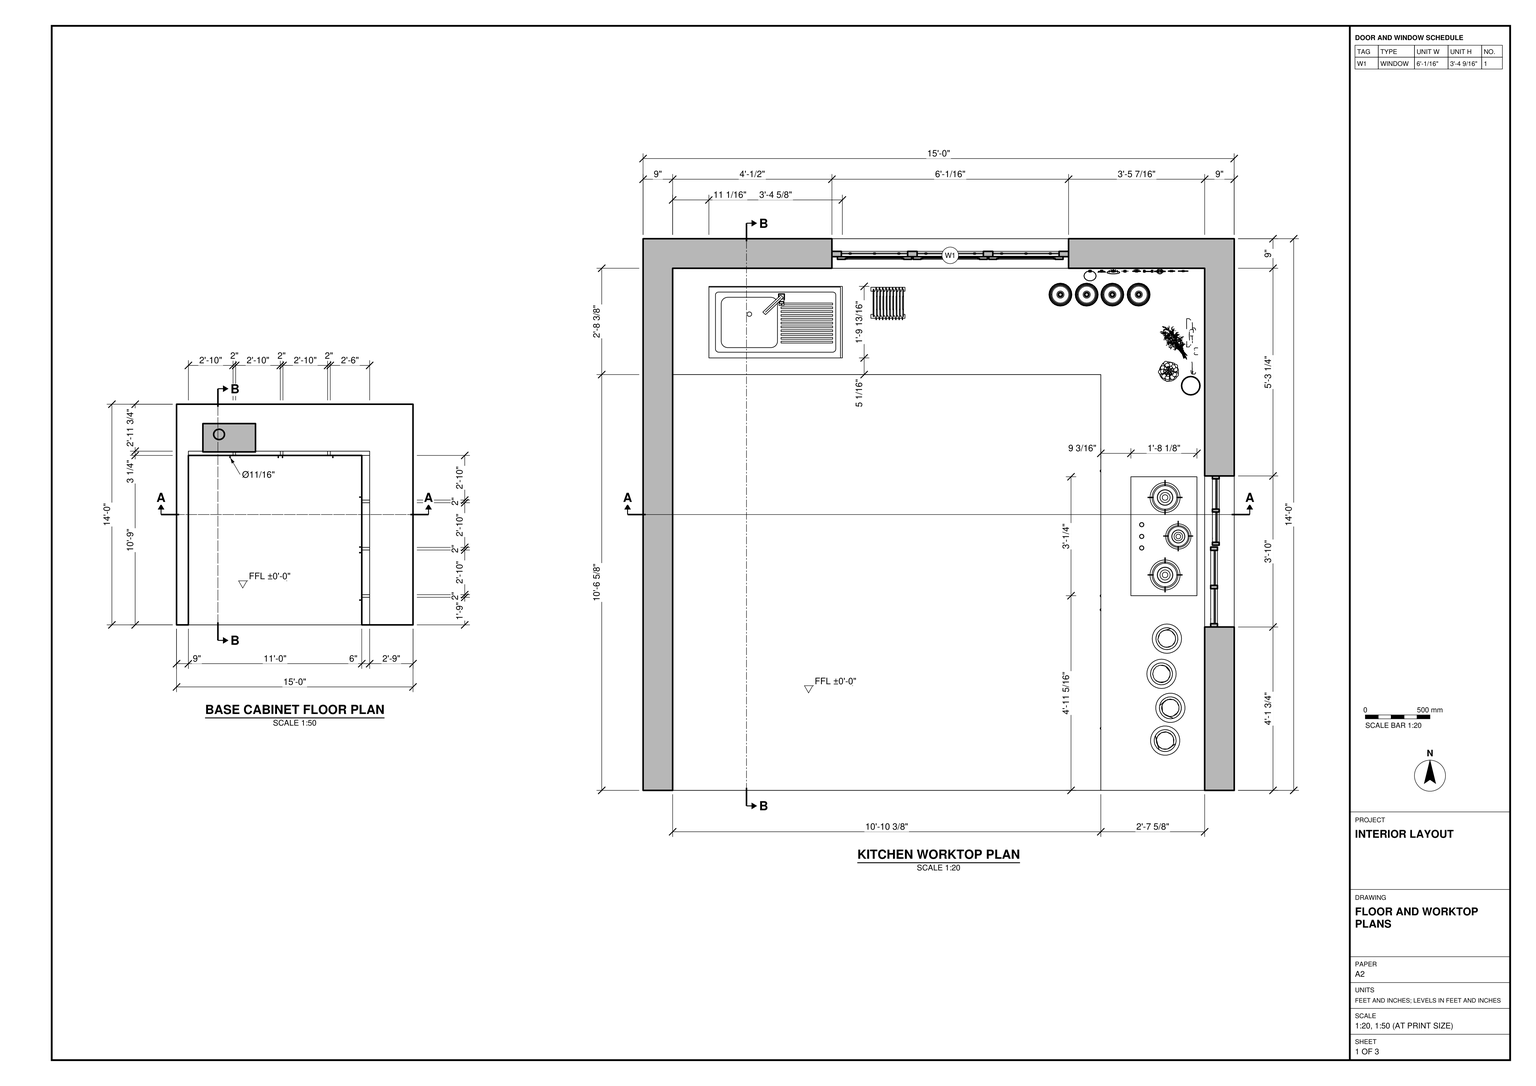
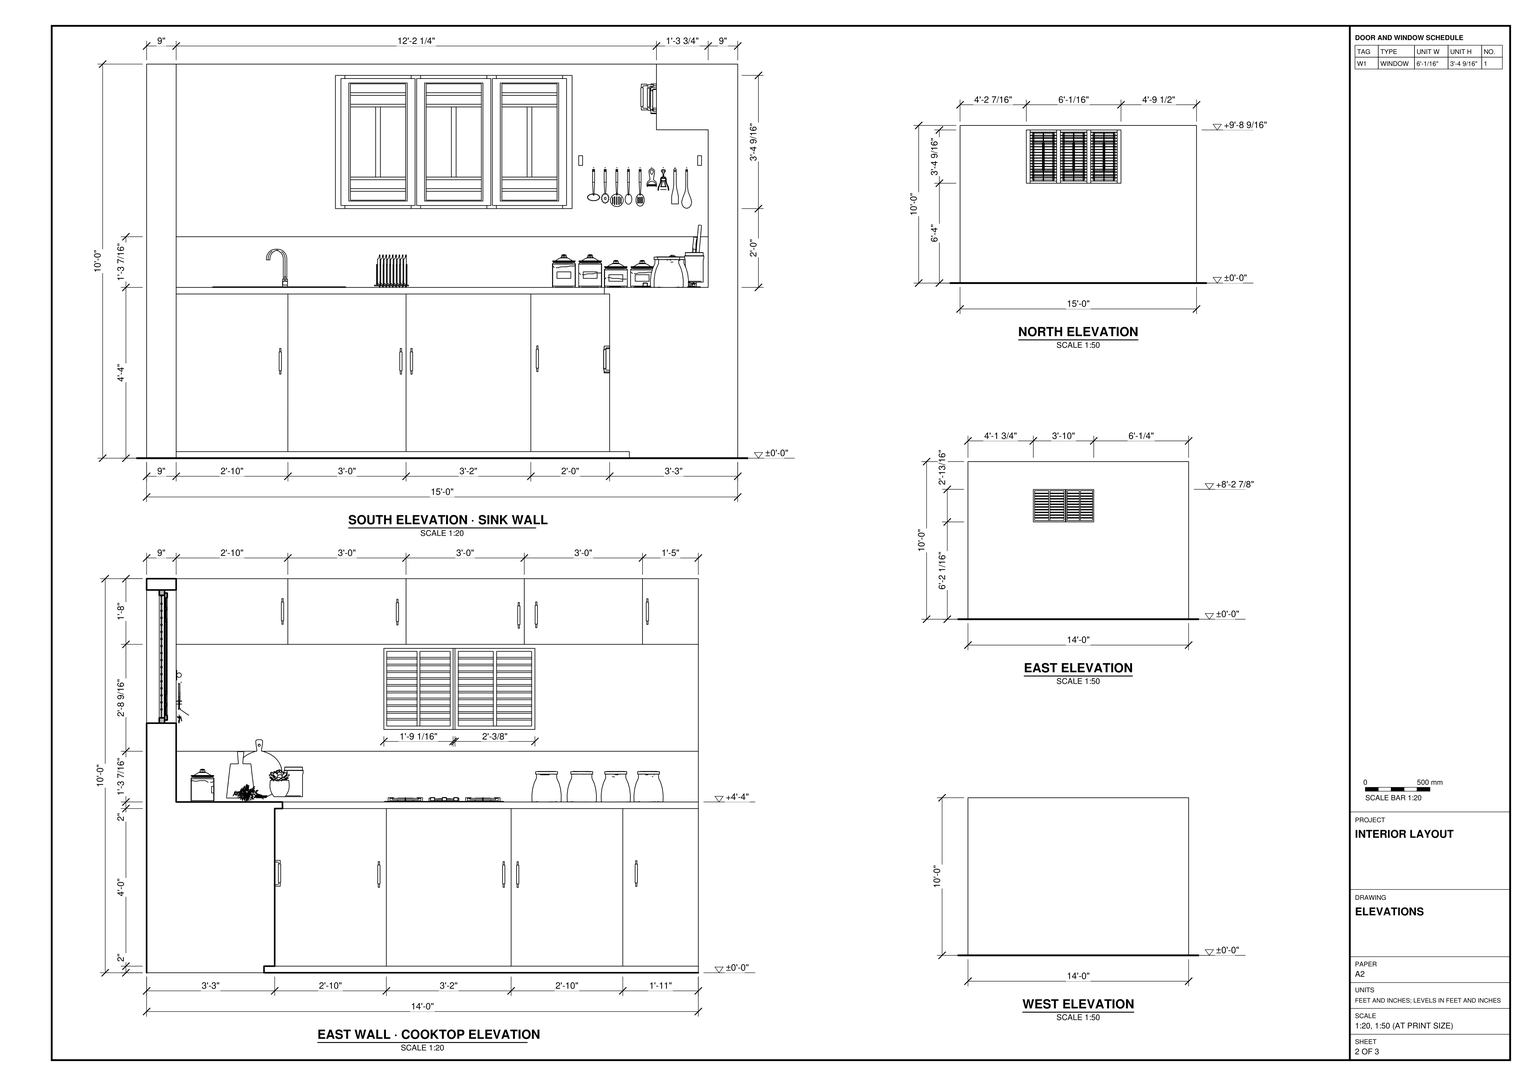
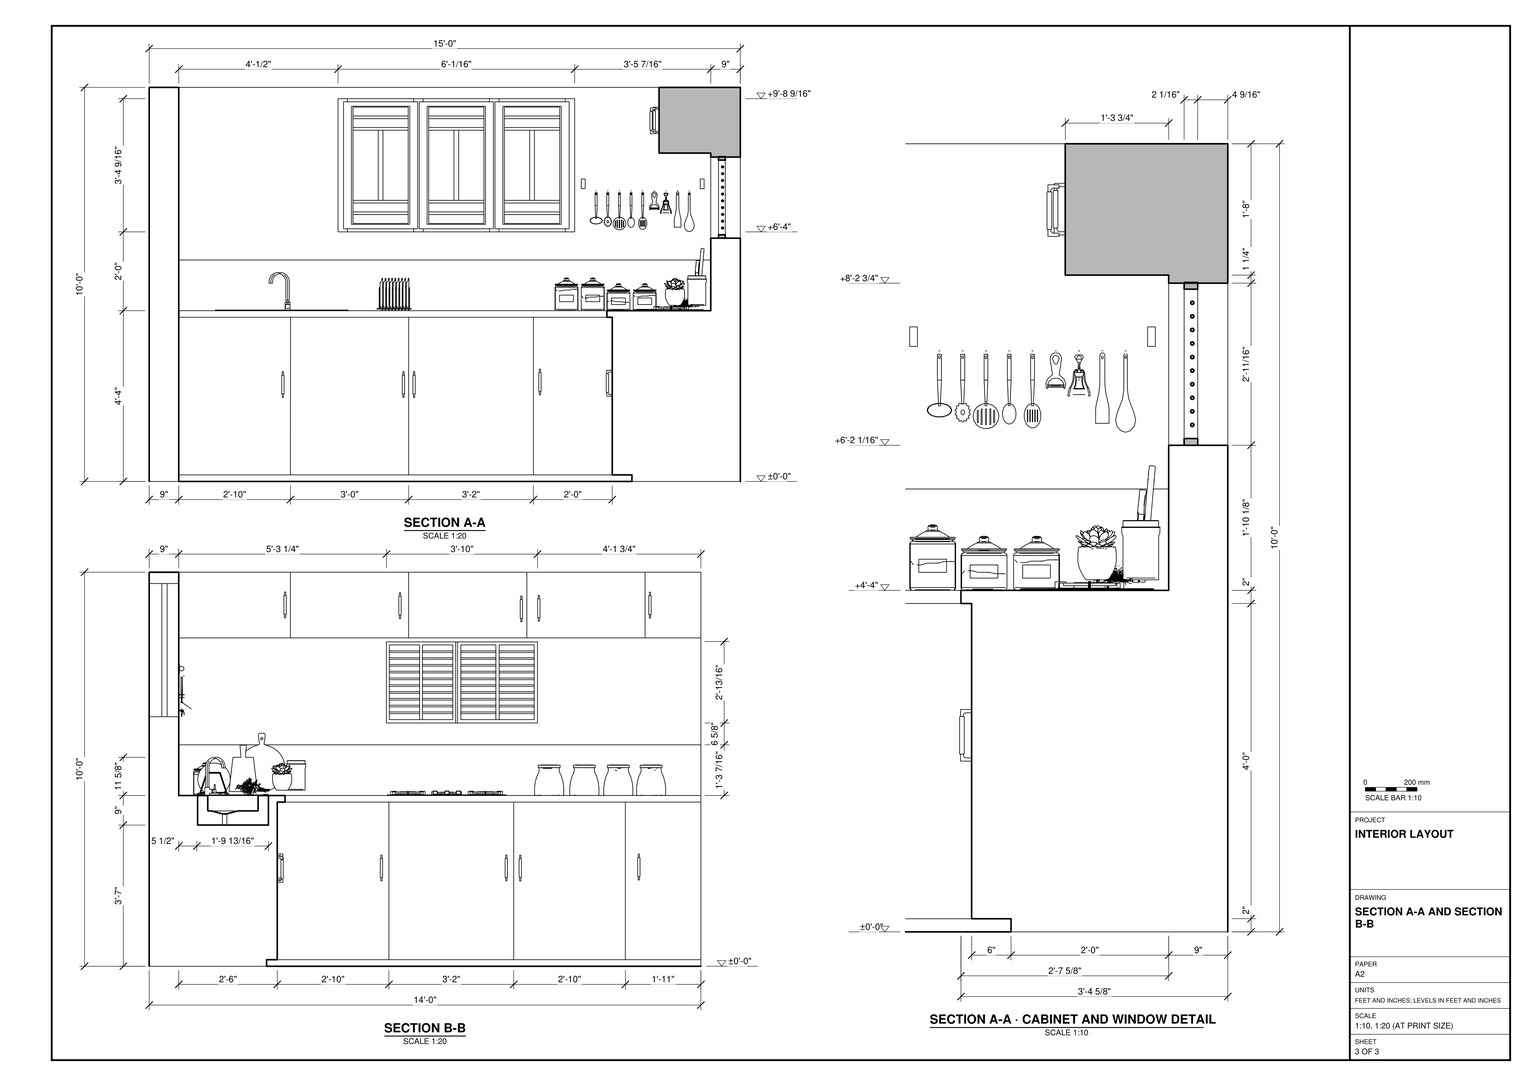
Build the kitchen interior in SketchUp from task_files/diagram_01.pdf. Work in feet and inches. Set the finished floor at ±0'-0" and make the overall model 15'-0" wide by 14'-0" deep by 10'-0" high. Model the floor and the 9" walls on the north, east and west sides, leaving the south side open as drawn. Use the plans to locate the openings and the elevations to set the sills and frames of the wide north window and smaller east window.

Fit a continuous L-shaped worktop along the north and east walls, with its top 4'-4" above the finished floor. Use the base cabinet plan for the cabinet divisions and the sections for the worktop edges and plinths. Place the sink toward the west end of the north run, with its tap and draining board, and fit the cooktop into the east return. Model the row of upper cabinets above the east window. Match the cabinet door widths and handle positions to the elevations.

Keep the floor, walls and each fitted joinery piece in separate groups or components, and use components for repeated parts. Decor, loose kitchen items and appliances may be any suitable library components placed as shown. Save one SketchUp model as output_files/l_shaped_kitchen_with_fitted_cabinets_and_window_units.skp.

# SketchUp Ruby script. Lengths in inches.
U = 1.inch
M = Sketchup.active_model
def pt(a) = Geom::Point3d.new(a.map { |v| v * U })
def face(e, loops, mat)
  f = e.add_face(loops[0].map { |a| pt(a) })
  loops[1..].each { |l| e.add_face(l.map { |a| pt(a) }).erase! }
  f.material = f.back_material = mat if mat
  f
end
# faces: each face lists its corners as indices into pts; further lists are holes
def faces(e, pts, list, mat = nil) = list.each { |f| face(e, (f[0].is_a?(Array) ? f : [f]).map { |l| l.map { |i| pts[i] } }, mat) }
# xy, xz, yz: faces in a plane at the given z, y or x. An outline is a flat list of corners, or four numbers for a rectangle; further outlines are holes
def ring(l) = l.size == 4 ? [[l[0], l[1]], [l[2], l[1]], [l[2], l[3]], [l[0], l[3]]] : l.each_slice(2).to_a
def flat(e, list, mat, &to3) = list.each { |f| face(e, (f[0].is_a?(Array) ? f : [f]).map { |l| ring(l).map { |u, v| to3.(u, v) } }, mat) }
def xy(e, z, list, mat = nil) = flat(e, list, mat) { |x, y| [x, y, z] }
def xz(e, y, list, mat = nil) = flat(e, list, mat) { |x, z| [x, y, z] }
def yz(e, x, list, mat = nil) = flat(e, list, mat) { |y, z| [x, y, z] }
def lines(e, pts, list) = list.each { |a, b| e.add_line(pt(pts[a]), pt(pts[b])) }
# prism: a flat outline (further loops are holes) pulled along v
def prism(e, loops, v, mat = nil)
  f = face(e, loops, mat); d = Geom::Vector3d.new(v.map { |x| x * U })
  f.pushpull(f.normal.samedirection?(d) ? d.length : -d.length)
end
def box(e, o, s, mat = nil) = prism(e, [[o, [o[0] + s[0], o[1], o[2]], [o[0] + s[0], o[1] + s[1], o[2]], [o[0], o[1] + s[1], o[2]]]], [0, 0, s[2]], mat)
def at(x, y, z, deg = 0) = Geom::Transformation.translation(pt([x, y, z])) * Geom::Transformation.rotation(ORIGIN, Z_AXIS, deg.degrees)
def axes(o, x, y, z) = Geom::Transformation.new([*x, 0, *y, 0, *z, 0, *pt(o).to_a, 1])
def part(name) = M.definitions.add(name)
# library, detail: a bought-in or finely detailed component or shape, given as its bounding box
def library(name, o, s) = part(name).tap { |d| box(d.entities, o, s) }
def detail(e, o, s) = box(e.add_group.entities, o, s)
def put(e, d, t, mat = nil) = e.add_instance(d, t).tap { |i| i.material = mat if mat }
def group(e, t, mat = nil) = e.add_group.tap { |g| g.transformation = t; g.material = mat if mat }.entities
root = M.entities
M.materials.add("[Cardboard]").color = [189, 139, 76]
M.materials.add("[Chipboard]").color = [205, 176, 119]
M.materials.add("[Color M08]").color = [30, 30, 30]
M.materials.add("[Encaustic Tile Circular 01]").color = [123, 123, 122]
M.materials.add("[Stone Vein Gray]").color = [166, 165, 165]
M.materials.add("[Translucent Glass Gray]").color = [128, 128, 128]
M.materials["[Translucent Glass Gray]"].alpha = 0.5
M.materials.add("[Wood Cherry Original]").color = [152, 86, 42]
M.materials.add("[Wood Floor Parquet]").color = [142, 87, 38]
M.materials.add("[Wood Veneer 01]").color = [120, 70, 37]
M.materials.add("[Wood Veneer 02]").color = [190, 128, 91]
c1 = library("w1.2X1.2",[0,0,0],[3.9375,47.24,47.24])
c2 = part("Group\#19")
box(c2.entities,[0,0,0],[13.78,1.18,1.18])
c3 = part("Group\#23")
box(c3.entities,[0,0.39,0],[13.78,0.4,3.9375])
c4 = part("Group\#21")
box(c4.entities,[0,0.39,0],[6.3,0.4,3.9375])
c5 = part("w3a")
g1 = group(c5.entities,at(-0.98,-1.18,-0.98),"[Wood Floor Parquet]")
xy(g1,0,[[0,0,18.5,1.18]])
xy(g1,1.97,[[1.97,0,16.54,0.39]])
xy(g1,2.36,[[2.36,0.39,16.14,1.18]])
xy(g1,53.9375,[[2.36,0.39,16.14,1.18]])
xy(g1,54.33,[[1.97,0,16.54,0.39]])
xy(g1,56.3,[[0,0,18.5,1.18]])
xz(g1,0,[[[0,0,18.5,56.3],[1.97,1.97,16.54,54.33]]])
xz(g1,0.39,[[[1.97,1.97,16.54,54.33],[2.36,2.36,16.14,53.9375]]])
xz(g1,1.18,[[[0,0,18.5,56.3],[2.36,2.36,16.14,53.9375]]])
yz(g1,0,[[0,0,1.18,56.3]])
yz(g1,1.97,[[0,1.97,0.39,54.33]])
yz(g1,2.36,[[0.39,2.36,1.18,53.9375]])
yz(g1,16.14,[[0.39,2.36,1.18,53.9375]])
yz(g1,16.54,[[0,1.97,0.39,54.33]])
yz(g1,18.5,[[0,0,1.18,56.3]])
g2 = group(c5.entities,at(1.38,-1.18,5.31),"[Wood Floor Parquet]")
put(g2,c2,axes([0,0.39,42.52],[1,0,0],[0,0.66667,0],[0,0,1]))
g3 = group(g2,at(6.3,0.39,20.08))
box(g3,[0,0,-13.78],[1.18,0.79,31.1])
put(g2,c2,axes([0,0.39,37.4],[1,0,0],[0,0.66667,0],[0,0,1]))
put(g2,c2,axes([0,0.39,0],[1,0,0],[0,0.66667,0],[0,0,1]))
put(g2,c2,axes([0,0.39,5.12],[1,0,0],[0,0.66667,0],[0,0,1]))
g4 = group(c5.entities,at(1.38,-0.39,1.38),"[Translucent Glass Gray]")
put(g4,c3,at(0,-0.39,5.12))
put(g4,c3,at(0,-0.39,0))
put(g4,c4,axes([0,-0.39,10.24],[1,0,0],[0,1,0],[0,0,7.9]))
put(g4,c4,axes([7.48,-0.39,10.24],[1,0,0],[0,1,0],[0,0,7.9]))
put(g4,c3,at(0,-0.39,47.64))
put(g4,c3,at(0,-0.39,42.52))
c6 = part("Group\#26")
box(c6.entities,[0,0,0],[0.39,0.39,54.33])
c7 = part("Group\#24")
box(c7.entities,[0,0,0],[0.39,0.39,5.68])
c8 = part("Group\#27")
box(c8.entities,[0,0,0],[0.39,0.39,2])
c9 = part("Group\#28")
put(c9.entities,c7,axes([14.14,0,0],[0,0,1],[0,1,0],[-1,0,0]))
put(c9.entities,c8,axes([2,0,0],[0,0,1],[0,1,0],[-1,0,0]))
put(c9.entities,c7,axes([8.07,0,0],[0,0,1],[0,1,0],[-1,0,0]))
put(c9.entities,c8,axes([16.54,0,0],[0,0,1],[0,1,0],[-1,0,0]))
c10 = part("Group\#29")
put(c10.entities,c6,at(12.15,0,0))
put(c10.entities,c6,at(6.07,0,0))
put(c10.entities,c6,at(0,0,0))
put(c10.entities,c9,at(-2,0,53.93))
put(c10.entities,c9,at(-2,0,50.39))
put(c10.entities,c9,at(-2,0,47.27))
put(c10.entities,c9,at(-2,0,44.14))
put(c10.entities,c9,at(-2,0,41.02))
put(c10.entities,c9,at(-2,0,37.9))
put(c10.entities,c9,at(-2,0,34.77))
put(c10.entities,c9,at(-2,0,31.65))
put(c10.entities,c9,at(-2,0,28.53))
put(c10.entities,c9,at(-2,0,25.4))
put(c10.entities,c9,at(-2,0,22.28))
put(c10.entities,c9,at(-2,0,19.16))
put(c10.entities,c9,at(-2,0,16.03))
put(c10.entities,c9,at(-2,0,12.91))
put(c10.entities,c9,at(-2,0,9.79))
put(c10.entities,c9,at(-2,0,6.66))
put(c10.entities,c9,at(-2,0,3.54))
c11 = part("Group\#16")
box(c11.entities,[0,0,0],[2.36,2.36,59.06])
c12 = part("Group\#1")
box(c12.entities,[0,0,0],[2.36,2.36,16.54])
c13 = part("W3")
put(c13.entities,c5,at(2.36,1.18,2.36))
put(c13.entities,c5,at(21.26,1.18,2.36))
put(c13.entities,c5,at(40.16,1.18,2.36))
put(c13.entities,c10,at(23.26,2.38,2.36),"[Color M08]")
put(c13.entities,c10,at(4.36,2.38,2.36),"[Color M08]")
put(c13.entities,c10,at(42.15,2.38,2.36),"[Color M08]")
g5 = group(c13.entities,at(0,1.18,0),"[Wood Veneer 01]")
put(g5,c11,at(0,0,0))
put(g5,c12,axes([2.36,0,2.36],[0,0,-1],[0,1,0],[1,0,0]))
put(g5,c11,at(18.9,0,0))
put(g5,c12,axes([21.26,0,2.36],[0,0,-1],[0,1,0],[1,0,0]))
put(g5,c11,at(37.8,0,0))
put(g5,c12,axes([40.16,0,2.36],[0,0,-1],[0,1,0],[1,0,0]))
put(g5,c11,at(56.69,0,0))
put(g5,c12,axes([2.36,0,59.06],[0,0,-1],[0,1,0],[1,0,0]))
put(g5,c12,axes([21.26,0,59.06],[0,0,-1],[0,1,0],[1,0,0]))
put(g5,c12,axes([40.16,0,59.06],[0,0,-1],[0,1,0],[1,0,0]))
c14 = part("Wooden+Window+W3")
put(c14.entities,c13,at(0,-1.18,35.43))
c15 = library("Cabinet pull handle",[0,0,0],[0.71,1.83,7.87])
c16 = library("Bosch Stove",[0,0,0],[36.22,20.12,1.38])
c17 = library("Component_12",[0,0,0],[17.72,31.5,20.63])
c18 = library("Plate rack",[-0.65,-0.94,-0.7],[10.38,9.93,9.93])
c19 = library("Glass_Apothecary_Jar",[-11.5,-3.52,0],[30.82,7.02,10])
c20 = library("ACCESS \#103",[-1.07,0,-1.17],[14.88,24.44,20.18])
c21 = library("Kitchen Utensils",[-18.7,-3.84,-14.5625],[37.4,3.84,16.04])
c22 = library("Group\#68",[0,0,0],[96.0625,96.0625,100.27])
c23 = library("Group\#67",[0,0,0],[96.0625,96.0625,100.24])
c24 = library("Group\#65",[0,0,0],[95.7,95.7,100.27])
c25 = library("Group\#64",[0,0,0],[95.7,95.7,100.27])
xy(root,0,[[9,0,147,132.25]])
xy(root,2,[[141,0,147,21],[141,21,147,23],[141,23,147,57],[141,57,147,59],[141,59,147,93],
  [141,93,147,95],[141,95,147,129],[9,129,43,132.25],[43,129,45,132.25],[45,129,79,132.25],
  [79,129,81,132.25],[81,129,115,132.25],[115,129,117,132.25],[117,129,147,132.25]])
xy(root,43,[[20.04,131.69,60.11,153.25]],"[Stone Vein Gray]")
xy(root,50,[[139.375,0,141,21],[139.375,21,141,57],[139.375,57,141,93],[139.375,93,139.375,126.625,117,126.625,117,129,141,129,141,93],[9,126.625,45,129],
  [45,126.625,81,129],[81,126.625,117,129]])
xy(root,52,[[[139.375,0,171,0,171,159,9,159,9,126.625,139.375,126.625],[20.04,131.69,60.11,153.25]]],"[Stone Vein Gray]")
xy(root,74.09,[[171,49.76,180,95.76]])
xy(root,76,[[57.49,159,129.56,168]])
xy(root,98.77,[[171,49.76,180,95.76]])
xy(root,100,[[155.25,0,171,15],[155.25,15,171,17],[155.25,17,171,51],[155.25,51,171,53],[155.25,53,171,87],
  [155.25,87,171,89],[155.25,89,171,123],[155.25,123,171,125],[155.25,125,171,159]])
xy(root,116.5625,[[57.49,159,129.56,168]])
xy(root,120,[[0,0,9,0,9,159,155.25,159,155.25,0,180,0,180,168,0,168]])
xz(root,0,[[0,0,9,120]])
xz(root,0,[[147,0,180,0,180,120,155.25,120,155.25,100,171,100,171,52,139.375,52,139.375,50,141,50,141,2,147,2]],"[Cardboard]")
xz(root,49.76,[[171,74.09,180,98.77]])
xz(root,95.76,[[171,74.09,180,98.77]])
xz(root,126.625,[[9,50,139.375,52]])
xz(root,129,[[9,2,43,2,43.03,50,9,50],[43,2,79,2,79,50,43.03,50],[79,2,117,50],[117,2,141,50]],"[Wood Cherry Original]")
xz(root,131.69,[[20.04,43,60.11,52]],"[Stone Vein Gray]")
xz(root,132.25,[[9,0,147,2]])
xz(root,153.25,[[20.04,43,60.11,52]],"[Stone Vein Gray]")
xz(root,159,[[[9,67.4375,171,67.4375,171,100,155.25,100,155.25,120,9,120],[57.49,76,129.56,116.5625]]])
xz(root,159,[[9,52,171,67.4375]],"[Encaustic Tile Circular 01]")
xz(root,168,[[[0,0,180,120],[57.49,76,129.56,116.5625]]])
yz(root,0,[[0,0,168,120]])
yz(root,9,[[0,0,132.25,0,132.25,2,129,2,129,50,126.625,50,126.625,52,159,52,159,120,0,120]],"[Chipboard]")
yz(root,20.04,[[131.69,43,153.25,52]],"[Stone Vein Gray]")
yz(root,57.49,[[159,76,168,116.5625]])
yz(root,60.11,[[131.69,43,153.25,52]],"[Stone Vein Gray]")
yz(root,129.56,[[159,76,168,116.5625]])
yz(root,139.375,[[0,50,126.625,52]])
yz(root,141,[[0,2,23,50],[23,2,57,50],[57,2,95,50],[95,2,129,50]],"[Wood Cherry Original]")
yz(root,147,[[0,0,132.25,2]])
yz(root,155.25,[[0,100,17,120],[17,100,53,120],[53,100,89,120],[89,100,125,120],[125,100,159,120]],"[Wood Veneer 02]")
yz(root,171,[[[0,67.4375,159,100],[49.76,74.09,95.76,98.77]]])
yz(root,171,[[0,52,159,67.4375]],"[Encaustic Tile Circular 01]")
yz(root,180,[[[0,0,168,120],[49.76,74.09,95.76,98.77]]])
put(root,c1,axes([173.35,74.67,74.09],[0.525,0,0],[0,0.44625,0],[0,0,0.525]))
put(root,c1,axes([172.83,49.76,74.09],[0.525,0,0],[0,0.51539,0],[0,0,0.525]))
put(root,c14,axes([57.49,162.52,51.66],[1.22026,0,0],[0,0.6868,0],[0,0,0.6868]))
put(root,c15,at(139.19,19.25,26.28,-90))
put(root,c15,at(139.15,55.36,25.96,-90))
put(root,c15,at(139.17,59.61,26,-90))
put(root,c15,at(139.17,97.625,26,-90))
put(root,c15,at(80.31,127.17,25.57))
put(root,c15,at(77.08,127.17,25.57))
put(root,c15,at(40.35,127.17,25.57))
put(root,c15,at(118.63,127.17,26.35))
put(root,c15,at(153.43,126.97,106.1,-90))
put(root,c15,at(152.48,91.98,105.89,-90))
put(root,c15,at(153.42,55.01,104.9,-90))
put(root,c15,at(153.42,49.69,105.09,-90))
put(root,c15,at(150.49,15.86,106.04,-90))
put(root,c16,at(148.53,95.51,52,-90))
put(root,c17,axes([20.04,153.48,43],[0,-1.23,0],[1.29,0,0],[0,0,1]))
put(root,c18,at(70.02,144.24,52.7))
put(root,c19,at(135.07,150.98,52))
put(root,c20,at(169.6875,143.68,52,180))
put(root,c21,at(150.27,159,90.63))
put(root,c22,axes([155.04,41.75,52],[0.0928,0,0],[0,0.0928,0],[0,0,0.0928]))
put(root,c23,axes([153.4,31.04,52],[0.0928,0,0],[0,0.0928,0],[0,0,0.0928]))
put(root,c24,axes([156.11,20.71,52],[0.0928,0,0],[0,0.0928,0],[0,0,0.0928]))
put(root,c25,axes([154.53,10.72,52],[0.0928,0,0],[0,0.0928,0],[0,0,0.0928]))
